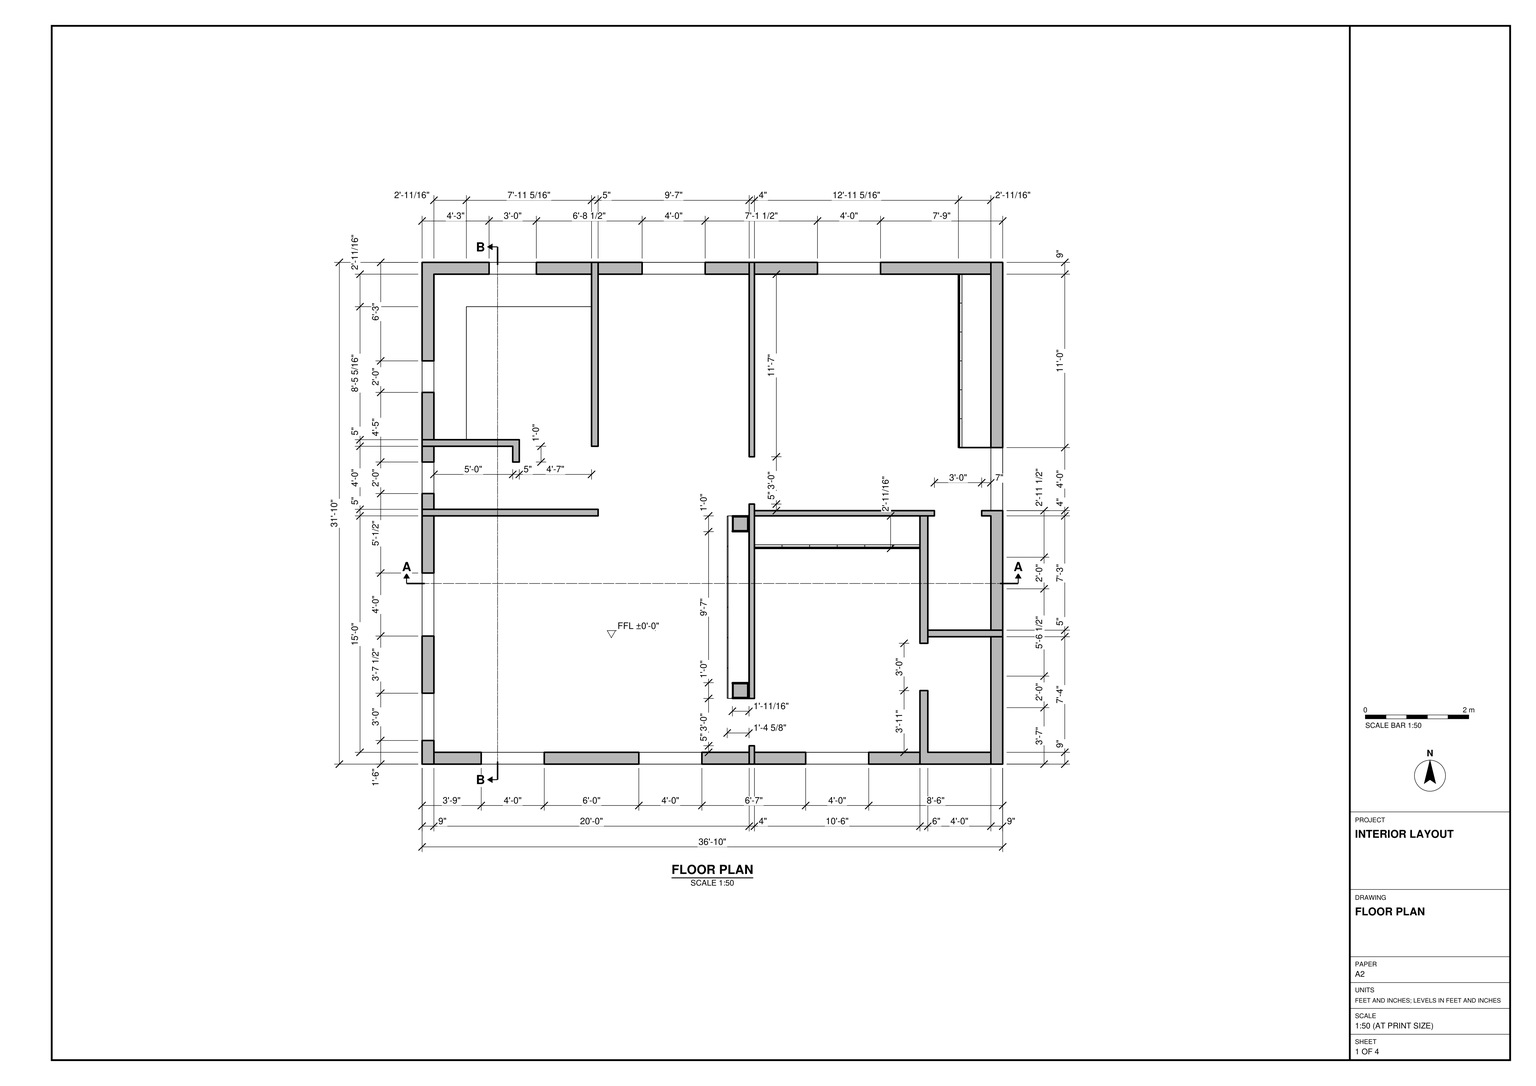
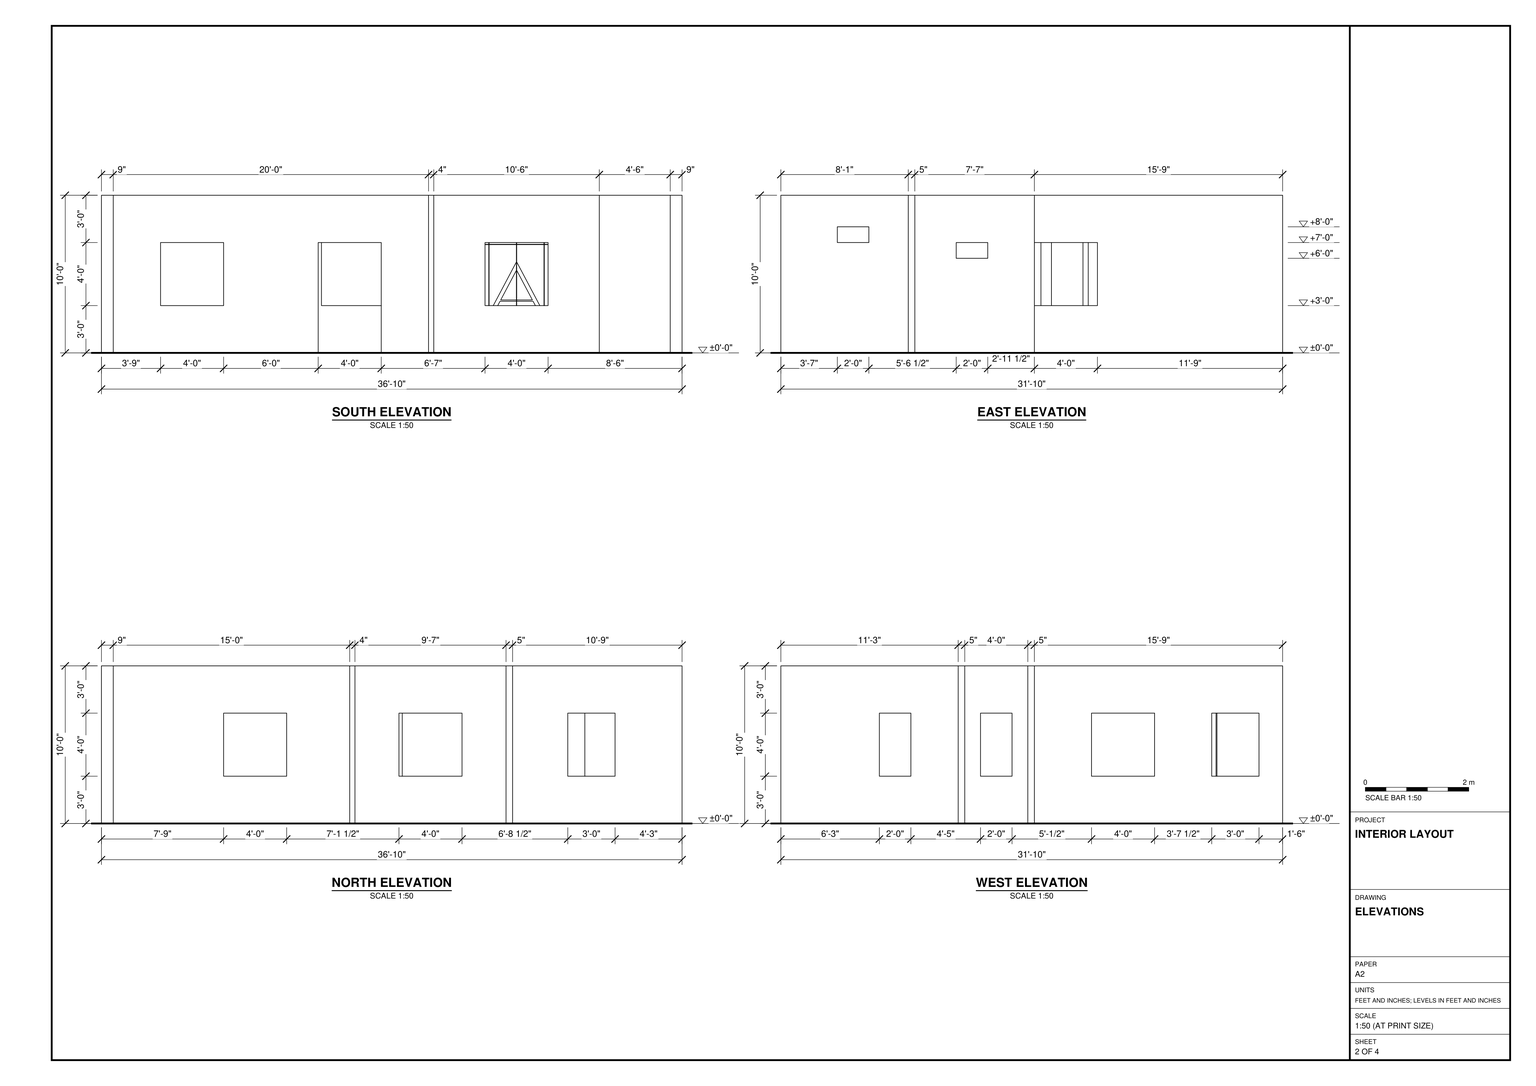
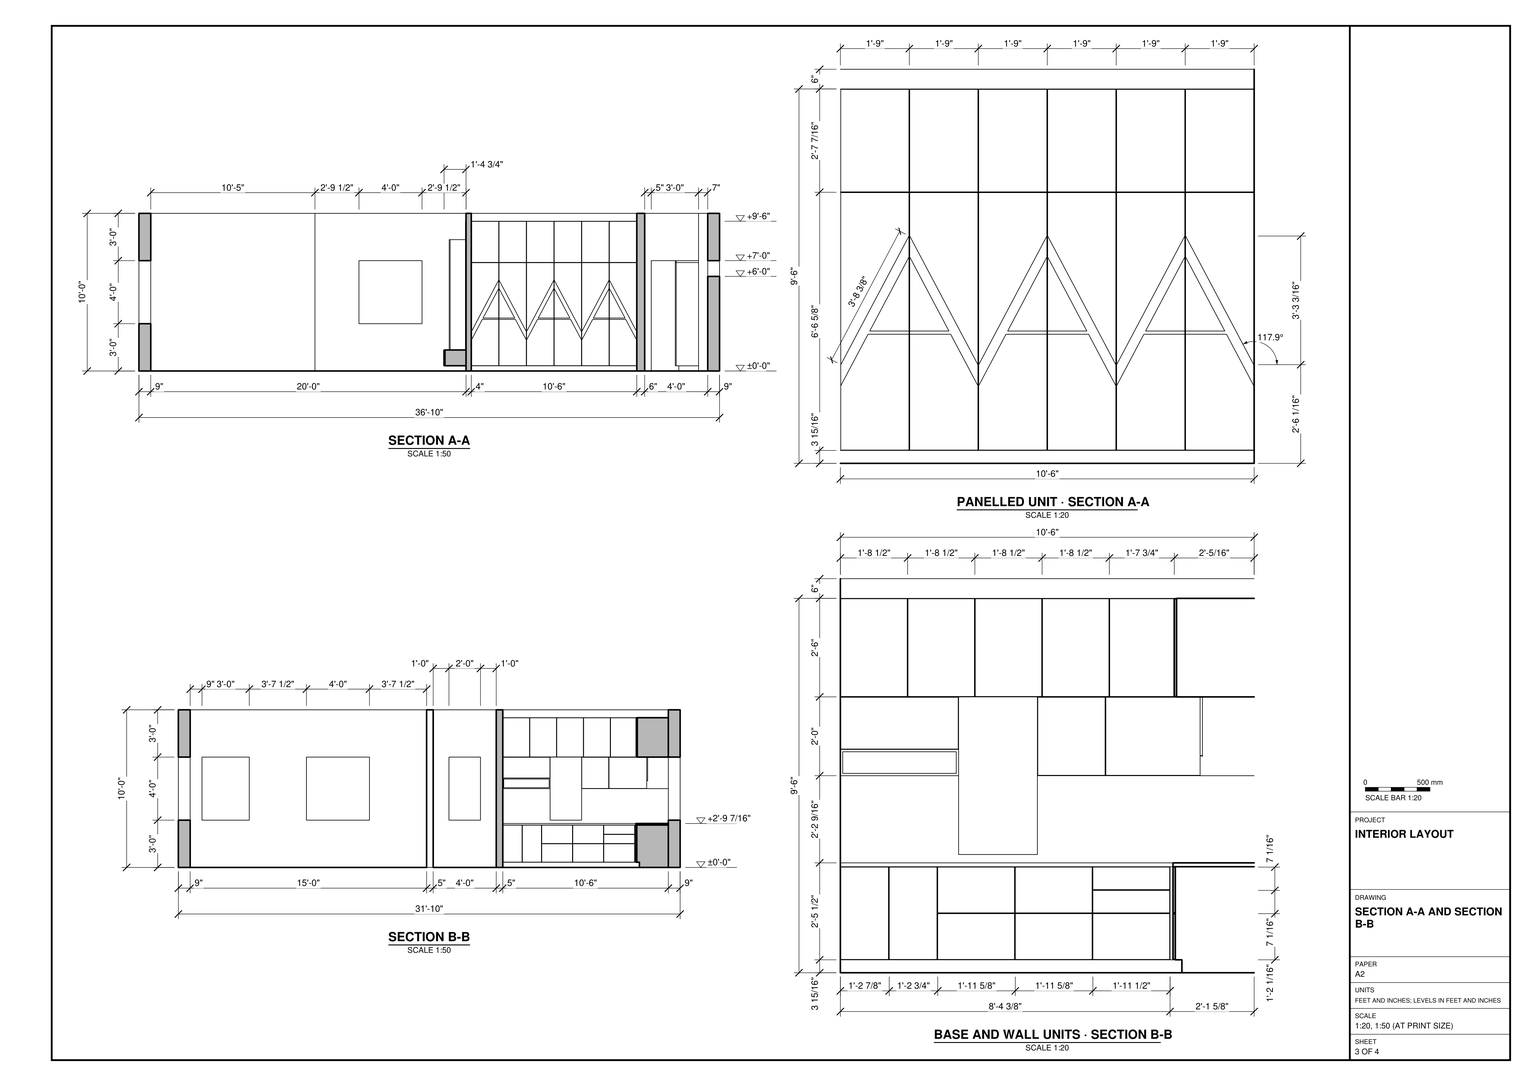
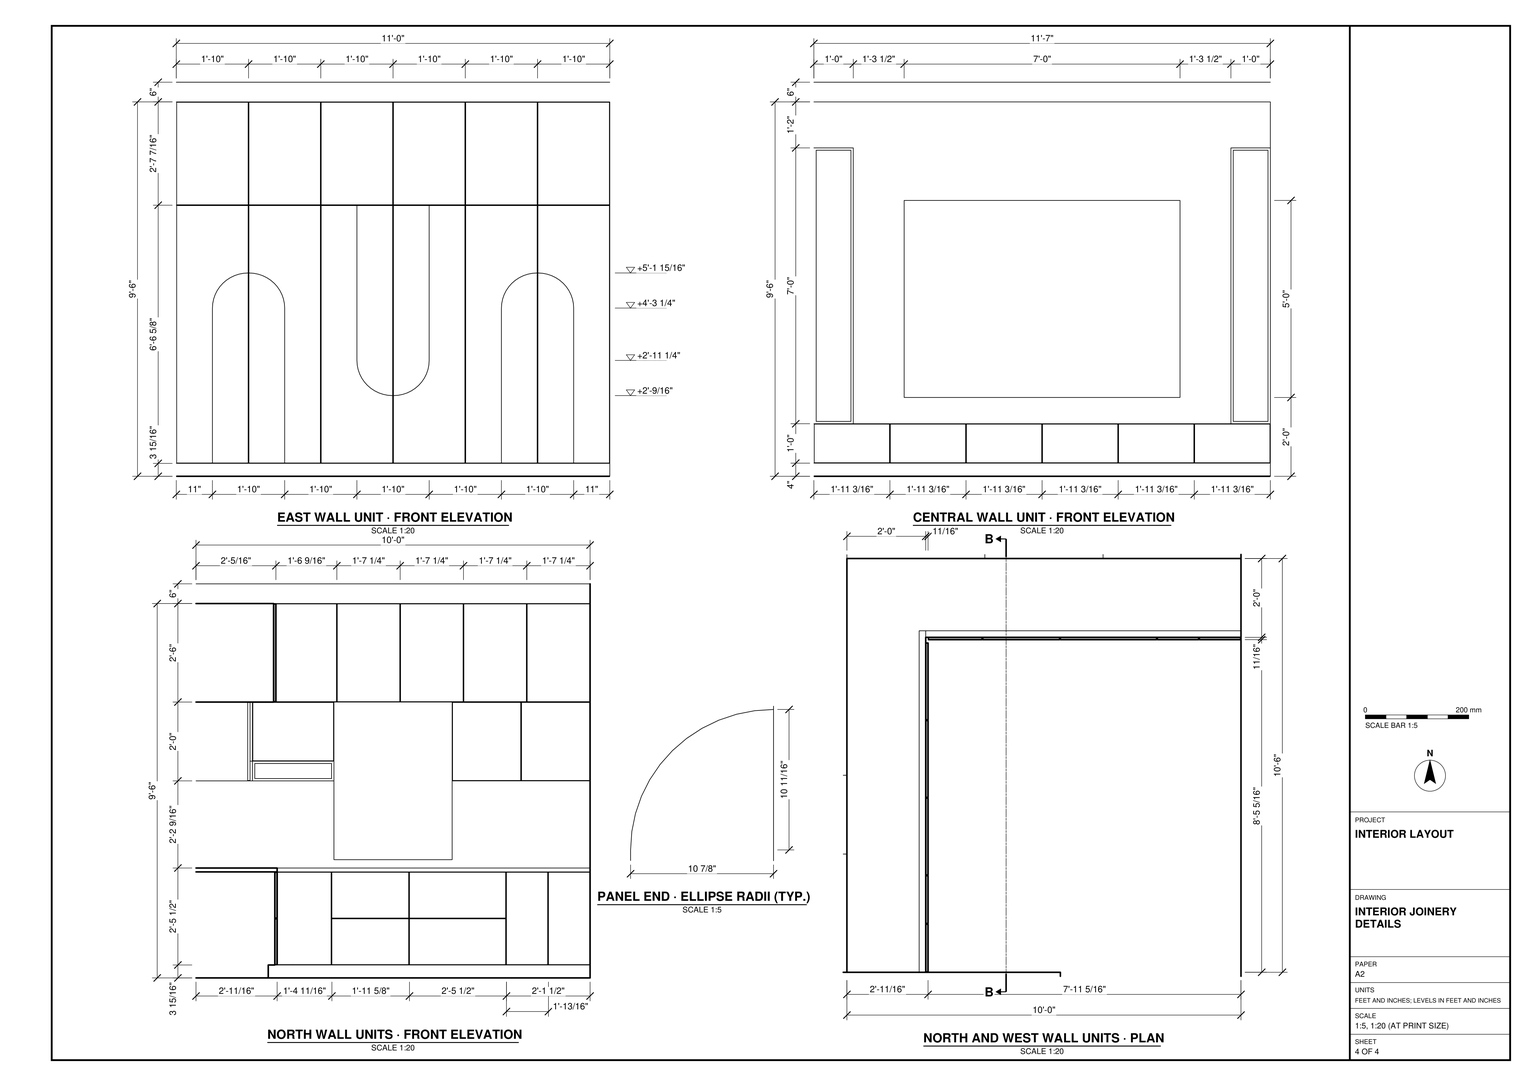
Build the interior in SketchUp using task_files/diagram_01.pdf. Work in feet and inches. Set the finished floor at ±0'-0" and lay out the rectangular shell at 36'-10" east to west by 31'-10" north to south, with an overall height of 10'-0".

Use the floor plan to locate the 9" perimeter walls and follow the individual thicknesses shown for the interior partitions. Preserve the passage between the northern bays and the southern rooms, including the short wall returns and the gaps between partition ends. Form the exterior openings through the walls. Use the elevations to set their widths, sills and heads, particularly the two small openings at different heights on the east wall.

Fit the panelled unit between the partitions shown in section A-A. Carry its three peaked motifs across the six vertical panels. For the cabinetry in section B-B, follow the enlarged detail for the base units, counter, upper cupboards and the spaces between them. Keep shell elements and each furniture or joinery piece in separate groups or components, and use components for repeated parts. Decor and loose items shown may be represented by any suitable library components. Save one SketchUp model as output_files/single_storey_interior_with_built_in_cabinetry.skp.

# SketchUp Ruby script. Lengths in inches.
U = 1.inch
M = Sketchup.active_model
def pt(a) = Geom::Point3d.new(a.map { |v| v * U })
def face(e, loops, mat)
  f = e.add_face(loops[0].map { |a| pt(a) })
  loops[1..].each { |l| e.add_face(l.map { |a| pt(a) }).erase! }
  f.material = f.back_material = mat if mat
  f
end
# faces: each face lists its corners as indices into pts; further lists are holes
def faces(e, pts, list, mat = nil) = list.each { |f| face(e, (f[0].is_a?(Array) ? f : [f]).map { |l| l.map { |i| pts[i] } }, mat) }
# xy, xz, yz: faces in a plane at the given z, y or x. An outline is a flat list of corners, or four numbers for a rectangle; further outlines are holes
def ring(l) = l.size == 4 ? [[l[0], l[1]], [l[2], l[1]], [l[2], l[3]], [l[0], l[3]]] : l.each_slice(2).to_a
def flat(e, list, mat, &to3) = list.each { |f| face(e, (f[0].is_a?(Array) ? f : [f]).map { |l| ring(l).map { |u, v| to3.(u, v) } }, mat) }
def xy(e, z, list, mat = nil) = flat(e, list, mat) { |x, y| [x, y, z] }
def xz(e, y, list, mat = nil) = flat(e, list, mat) { |x, z| [x, y, z] }
def yz(e, x, list, mat = nil) = flat(e, list, mat) { |y, z| [x, y, z] }
def lines(e, pts, list) = list.each { |a, b| e.add_line(pt(pts[a]), pt(pts[b])) }
# prism: a flat outline (further loops are holes) pulled along v
def prism(e, loops, v, mat = nil)
  f = face(e, loops, mat); d = Geom::Vector3d.new(v.map { |x| x * U })
  f.pushpull(f.normal.samedirection?(d) ? d.length : -d.length)
end
def box(e, o, s, mat = nil) = prism(e, [[o, [o[0] + s[0], o[1], o[2]], [o[0] + s[0], o[1] + s[1], o[2]], [o[0], o[1] + s[1], o[2]]]], [0, 0, s[2]], mat)
def at(x, y, z, deg = 0) = Geom::Transformation.translation(pt([x, y, z])) * Geom::Transformation.rotation(ORIGIN, Z_AXIS, deg.degrees)
def axes(o, x, y, z) = Geom::Transformation.new([*x, 0, *y, 0, *z, 0, *pt(o).to_a, 1])
def part(name) = M.definitions.add(name)
# library, detail: a bought-in or finely detailed component or shape, given as its bounding box
def library(name, o, s) = part(name).tap { |d| box(d.entities, o, s) }
def detail(e, o, s) = box(e.add_group.entities, o, s)
def put(e, d, t, mat = nil) = e.add_instance(d, t).tap { |i| i.material = mat if mat }
def group(e, t, mat = nil) = e.add_group.tap { |g| g.transformation = t; g.material = mat if mat }.entities
root = M.entities
M.materials.add("[0006_Pink]").color = [206, 155, 164]
M.materials.add("[0009_Linen]").color = [234, 225, 215]
M.materials.add("[0053_Ivory]").color = [255, 255, 240]
M.materials.add("[0128_White]").color = [255, 255, 255]
M.materials.add("[0129_WhiteSmoke]").color = [237, 237, 237]
M.materials.add("[0132_LightGray]").color = [234, 234, 234]
M.materials.add("[Translucent Glass Gray]").color = [128, 128, 128]
M.materials["[Translucent Glass Gray]"].alpha = 0.5
M.materials.add("[Wood Cherry Original]").color = [152, 86, 42]
c1 = part("Group\#22")
xy(c1.entities,0.12,[[0,0.12,0.71,21.88]])
xy(c1.entities,31.88,[[0,0.12,0.71,21.88]])
xz(c1.entities,0.12,[[0,0.12,0.71,31.88]])
xz(c1.entities,21.88,[[0,0.12,0.71,31.88]])
yz(c1.entities,0,[[0.12,0.12,21.88,31.88]])
yz(c1.entities,0.71,[[[0,0,22,32],[0.12,0.12,21.88,31.88]]])
c2 = part("Group\#51")
xy(c2.entities,0.12,[[0.12,0,20.88,0.71]])
xy(c2.entities,31.88,[[0.12,0,20.88,0.71]])
xz(c2.entities,0,[[0.12,0.12,20.88,31.88]])
xz(c2.entities,0.71,[[[0,0,21,32],[0.12,0.12,20.88,31.88]]])
yz(c2.entities,0.12,[[0,0.12,0.71,31.88]])
yz(c2.entities,20.88,[[0,0.12,0.71,31.88]])
c3 = part("Group\#31")
xy(c3.entities,0.12,[[0.12,0,19.16,0.71]])
xy(c3.entities,29.88,[[0.12,0,19.16,0.71]])
xz(c3.entities,0,[[0.12,0.12,19.16,29.88]])
xz(c3.entities,0.71,[[[0,0,19.28,30],[0.12,0.12,19.16,29.88]]])
yz(c3.entities,0.12,[[0,0.12,0.71,29.88]])
yz(c3.entities,19.16,[[0,0.12,0.71,29.88]])
c4 = part("Group\#32")
xy(c4.entities,0.12,[[0,0.12,0.71,20.36]])
xy(c4.entities,29.88,[[0,0.12,0.71,20.36]])
xz(c4.entities,0.12,[[0,0.12,0.71,29.88]])
xz(c4.entities,20.36,[[0,0.12,0.71,29.88]])
yz(c4.entities,0,[[[0,0,20.48,30],[0.12,0.12,20.36,29.88]]])
yz(c4.entities,0.71,[[0.12,0.12,20.36,29.88]])
c5 = part("Group\#38")
xy(c5.entities,0,[[0,0,12,12]])
xy(c5.entities,0.71,[[0,0.71,11,11.29]])
xy(c5.entities,14.47,[[0,0.71,11,11.29]])
xy(c5.entities,15.18,[[0,0.71,11,11.29]])
xy(c5.entities,28.24,[[0,0.71,11,11.29]])
xy(c5.entities,28.94,[[0,0.71,11,11.29]])
xy(c5.entities,42,[[0,0.71,11,11.29]])
xy(c5.entities,42.71,[[0,0.71,11,11.29]])
xy(c5.entities,55.76,[[0,0.71,11,11.29]])
xy(c5.entities,56.47,[[0,0.71,11,11.29]])
xy(c5.entities,69.53,[[0,0.71,11,11.29]])
xy(c5.entities,70.24,[[0,0.71,11,11.29]])
xy(c5.entities,83.29,[[0,0.71,11,11.29]])
xy(c5.entities,84,[[0,0,12,12]])
xz(c5.entities,0,[[0,0,12,84]])
xz(c5.entities,0.71,[[0,0.71,11,14.47],[0,15.18,11,28.24],[0,28.94,11,42],[0,42.71,11,55.76],[0,56.47,11,69.53],
  [0,70.24,11,83.29]])
xz(c5.entities,11.29,[[0,0.71,11,14.47],[0,15.18,11,28.24],[0,28.94,11,42],[0,42.71,11,55.76],[0,56.47,11,69.53],
  [0,70.24,11,83.29]])
xz(c5.entities,12,[[0,0,12,84]])
yz(c5.entities,0,[[[0,0,12,84],[0.71,0.71,11.29,83.29]],[0.71,14.47,11.29,15.18],[0.71,28.24,11.29,28.94],[0.71,42,11.29,42.71],[0.71,55.76,11.29,56.47],
  [0.71,69.53,11.29,70.24]])
yz(c5.entities,11,[[0.71,0.71,11.29,14.47],[0.71,15.18,11.29,28.24],[0.71,28.94,11.29,42],[0.71,42.71,11.29,55.76],[0.71,56.47,11.29,69.53],
  [0.71,70.24,11.29,83.29]])
yz(c5.entities,12,[[0,0,12,84]])
g1 = group(c5.entities,at(-0.71,0,0))
prism(g1,[[[0.71,0,0],[0.71,12,0],[0.71,12,84],[0.71,0,84]],[[0.71,11.29,0.71],[0.71,0.71,0.71],[0.71,0.71,83.29],[0.71,11.29,83.29]]],[-0.71,0,0])
g2 = group(g1,at(0.2,0.71,0.71),"[Translucent Glass Gray]")
box(g2,[0,0,0],[0.31,10.58,82.58])
c6 = part("Group\#41")
xy(c6.entities,0.12,[[0,0.12,0.71,23.05]])
xy(c6.entities,11.88,[[0,0.12,0.71,23.05]])
xz(c6.entities,0.12,[[0,0.12,0.71,11.88]])
xz(c6.entities,23.05,[[0,0.12,0.71,11.88]])
yz(c6.entities,0,[[0.12,0.12,23.05,11.88]])
yz(c6.entities,0.71,[[[0,0,23.17,12],[0.12,0.12,23.05,11.88]]])
xy(root,0,[[45,0,93,9],[129,0,165,9],[165,0,225,9],[292,0,340,9],[9,9,249,9,249,14,253,14,253,9,379,9,379,56,385,56,385,9,433,9,433,97,385,97,385,92,379,92,379,189,253,189,253,50,249,50,249,198,253,198,253,193,390,193,390,189,385,189,385,102,433,102,433,189,426,189,426,193,433,193,433,373,253,373,253,234,249,234,249,373,134,373,134,242,129,242,129,373,9,373,9,247,74,247,74,230,69,230,69,242,9,242,9,194,134,194,134,189,9,189],
  [0,18,9,54],[433,43,442,67],[0,97.5,9,145.5],[433,133.5,442,157.5],[433,193,442,241],
  [0,206,9,230],[0,283,9,307],[51,373,87,382],[167.5,373,215.5,382],[301,373,349,382]])
xy(root,120,[[0,189,134,194]],"[0132_LightGray]")
xz(root,189,[[0,0,134,120]],"[0132_LightGray]")
xz(root,194,[[0,0,9,120],[9,0,134,120]])
yz(root,0,[[189,0,194,120]],"[0132_LightGray]")
yz(root,134,[[189,0,194,120]])
g3 = group(root,at(0,247,0),"[0132_LightGray]")
xy(g3,0,[[0,0,9,36],[0,36,9,135],[9,126,87,135],[87,126,129,135]])
xy(g3,36,[[0,36,9,60],[51,126,87,135]])
xy(g3,84,[[0,36,9,60],[51,126,87,135]])
xy(g3,120,[[0,0,9,0,9,126,129,126,129,135,0,135]])
xz(g3,0,[[0,0,9,120]])
xz(g3,36,[[0,36,9,84]])
xz(g3,60,[[0,36,9,84]])
xz(g3,126,[[[9,0,129,120],[51,36,87,84]]])
xz(g3,135,[[[0,0,129,120],[51,36,87,84]]])
yz(g3,0,[[[0,0,135,120],[36,36,60,84]]])
yz(g3,9,[[[0,0,126,120],[36,36,60,84]]])
yz(g3,51,[[126,36,135,84]])
yz(g3,87,[[126,36,135,84]])
yz(g3,129,[[126,0,135,120]])
g4 = group(root,at(0,230,0),"[0132_LightGray]")
xy(g4,0,[[69,0,69,12,0,12,0,17,74,17,74,0]])
xy(g4,84,[[69,-36,74,0]])
xy(g4,120,[[69,-36,74,-36,74,17,0,17,0,12,69,12]])
xz(g4,-36,[[69,84,74,120]])
xz(g4,0,[[69,0,74,84]])
xz(g4,12,[[0,0,69,120]])
xz(g4,17,[[0,0,9,120],[9,0,74,120]])
yz(g4,0,[[12,0,17,120]])
yz(g4,69,[[0,0,0,84,-36,84,-36,120,12,120,12,0]])
yz(g4,74,[[0,0,17,0,17,120,-36,120,-36,84,0,84]])
g5 = group(root,at(0,194,0),"[0132_LightGray]")
prism(g5,[[[9,48,120],[9,0,120],[9,0,0],[9,12,0],[9,48,0]],[[9,12,36],[9,12,84],[9,36,84],[9,36,36]]],[-9,0,0])
g6 = group(root,at(0,0,0),"[0132_LightGray]")
prism(g6,[[[9,0,0],[9,18,0],[9,97.5,0],[9,189,0],[9,189,120],[9,0,120]],[[9,97.5,36],[9,97.5,84],[9,145.5,84],[9,145.5,36]],[[9,54,36],[9,18,36],[9,18,84],[9,54,84]]],[-9,0,0])
g7 = group(root,at(9,0,0),"[0132_LightGray]")
prism(g7,[[[240,9,0],[204,9,0],[204,9,84],[156,9,84],[156,9,0],[84,9,0],[0,9,0],[0,9,120],[240,9,120]],[[36,9,36],[84,9,36],[84,9,84],[36,9,84]]],[0,-9,0])
g8 = group(root,at(249,0,0),"[0132_LightGray]")
xy(g8,0,[[0,0,4,14],[0,50,4,198]])
xy(g8,84,[[0,14,4,50]])
xy(g8,120,[[0,0,4,198]])
xz(g8,0,[[0,0,4,120]])
xz(g8,14,[[0,0,4,84]])
xz(g8,50,[[0,0,4,84]])
xz(g8,198,[[0,0,4,120]])
yz(g8,0,[[0,0,9,120],[9,0,9,120,198,120,198,0,50,0,50,84,14,84,14,0]])
yz(g8,4,[[0,0,14,0,14,84,50,84,50,0,198,0,198,120,0,120]])
g9 = group(root,at(253,0,0),"[0132_LightGray]")
prism(g9,[[[126,9,0],[87,9,0],[0,9,0],[0,9,120],[126,9,120]],[[39,9,36],[87,9,36],[87,9,84],[39,9,84]]],[0,-9,0])
g10 = group(root,at(379,0,0),"[0132_LightGray]")
xy(g10,0,[[0,0,6,56],[6,0,54,9]])
xy(g10,84,[[0,56,6,92]])
xy(g10,120,[[0,0,54,0,54,9,6,9,6,92,0,92]])
xz(g10,0,[[0,0,54,120]])
xz(g10,9,[[6,0,54,120]])
xz(g10,56,[[0,0,6,84]])
xz(g10,92,[[0,84,6,120]])
yz(g10,0,[[0,0,9,120],[9,0,9,120,92,120,92,84,56,84,56,0]])
yz(g10,6,[[9,0,56,0,56,84,92,84,92,120,9,120]])
yz(g10,54,[[0,0,9,120]])
g11 = group(root,at(433,0,0),"[0132_LightGray]")
xy(g11,0,[[0,0,9,67],[0,67,9,97]])
xy(g11,84,[[0,43,9,67]])
xy(g11,96,[[0,43,9,67]])
xy(g11,120,[[0,0,9,97]])
xz(g11,0,[[0,0,9,120]])
xz(g11,43,[[0,84,9,96]])
xz(g11,67,[[0,84,9,96]])
xz(g11,97,[[0,0,9,120]])
yz(g11,0,[[0,0,9,120],[[9,0,97,120],[43,84,67,96]]])
yz(g11,9,[[[0,0,97,120],[43,84,67,96]]])
g12 = group(root,at(385,97,0),"[0132_LightGray]")
prism(g12,[[[48,0,0],[0,0,0],[0,5,0],[57,5,0],[57,0,0]]],[0,0,120])
g13 = group(root,at(426,102,0),"[0132_LightGray]")
xy(g13,0,[[7,0,16,55.5],[7,55.5,7,87,0,87,0,91,16,91,16,55.5]])
xy(g13,72,[[7,31.5,16,55.5]])
xy(g13,84,[[7,31.5,16,55.5]])
xy(g13,120,[[7,0,16,0,16,91,0,91,0,87,7,87]])
xz(g13,0,[[7,0,16,120]])
xz(g13,31.5,[[7,72,16,84]])
xz(g13,55.5,[[7,72,16,84]])
xz(g13,87,[[0,0,7,120]])
xz(g13,91,[[0,0,16,120]])
yz(g13,0,[[87,0,91,120]])
yz(g13,7,[[[0,0,87,120],[31.5,72,55.5,84]]])
yz(g13,16,[[[0,0,91,120],[31.5,72,55.5,84]]])
g14 = group(root,at(379,92,0),"[0132_LightGray]")
prism(g14,[[[0,0,0],[0,97,0],[6,97,0],[6,10,0],[6,5,0],[6,0,0]]],[0,0,120])
g15 = group(root,at(253,189,0),"[0132_LightGray]")
xy(g15,0,[[0,0,137,4]])
xy(g15,84,[[137,0,173,4]])
xy(g15,120,[[0,0,173,4]])
xz(g15,0,[[0,0,126,120],[126,0,132,120],[132,0,137,0,137,84,173,84,173,120,132,120]])
xz(g15,4,[[0,0,0,120,173,120,173,84,137,84,137,0]])
yz(g15,0,[[0,0,4,120]])
yz(g15,137,[[0,0,4,84]])
yz(g15,173,[[0,84,4,120]])
g16 = group(root,at(433,241,0),"[0132_LightGray]")
prism(g16,[[[0,-48,84],[0,-48,120],[0,141,120],[0,141,0],[0,-48,0],[0,-48,36],[0,0,36],[0,0,84]]],[9,0,0])
g17 = group(root,at(129,242,0),"[0132_LightGray]")
prism(g17,[[[5,140,0],[5,0,0],[0,0,0],[0,131,0],[0,140,0]]],[0,0,120])
g18 = group(root,at(134,373,0),"[0132_LightGray]")
prism(g18,[[[115,0,0],[115,0,120],[0,0,120],[0,0,0],[33.5,0,0]],[[33.5,0,36],[33.5,0,84],[81.5,0,84],[81.5,0,36]]],[0,9,0])
g19 = group(root,at(249,234,0),"[0132_LightGray]")
xy(g19,0,[[0,0,4,148]])
xy(g19,84,[[0,-36,4,0]])
xy(g19,120,[[0,-36,4,148]])
xz(g19,-36,[[0,84,4,120]])
xz(g19,0,[[0,0,4,84]])
xz(g19,148,[[0,0,4,120]])
yz(g19,0,[[0,0,0,84,-36,84,-36,120,139,120,139,0],[139,0,148,120]])
yz(g19,4,[[0,0,148,0,148,120,-36,120,-36,84,0,84]])
g20 = group(root,at(253,373,0),"[0132_LightGray]")
prism(g20,[[[180,9,0],[96,9,0],[0,9,0],[0,9,120],[180,9,120]],[[48,9,36],[96,9,36],[96,9,84],[48,9,84]]],[0,-9,0])
g21 = group(root,at(409,234,0),"[0009_Linen]")
xy(g21,0,[[2,7,24,139]])
xy(g21,3.93,[[0,7,2,29],[2,7,24,139],[0,29,2,51],[0,51,2,73],[0,73,2,95],
  [0,95,2,117],[0,117,2,139]])
xy(g21,82.55,[[0,7,24,139]])
xy(g21,114,[[0,7,24,139]])
xz(g21,7,[[2,0,24,3.93],[0,3.93,24,82.55],[0,82.55,24,114]])
xz(g21,139,[[2,0,24,3.93],[0,3.93,24,82.55],[0,82.55,24,114]])
yz(g21,0,[[7,3.93,29,82.55],[29,3.93,51,82.55],[51,3.93,73,82.55],[73,3.93,95,82.55],[95,3.93,117,82.55],
  [117,3.93,139,82.55],[7,82.55,29,114],[29,82.55,51,114],[51,82.55,73,114],[73,82.55,95,114],
  [95,82.55,117,114],[117,82.55,139,114]])
yz(g21,2,[[7,0,139,3.93]])
yz(g21,24,[[7,0,139,3.93],[7,3.93,139,82.55],[7,82.55,139,114]])
g22 = group(g21,at(-0.71,29,3.93))
xy(g22,0.12,[[0,0.12,0.71,21.88]])
xy(g22,78.5,[[0,0.12,0.71,21.88]])
xz(g22,0.12,[[0,0.12,0.71,78.5]])
xz(g22,21.88,[[0,0.12,0.71,78.5]])
yz(g22,0,[[11,0.12,11,47.29,10.91,48.68,10.63,50.06,10.17,51.38,9.54,52.64,8.75,53.8,7.8125,54.85,6.74,55.77,5.56,56.55,4.28,57.17,2.93,57.62,1.54,57.89,0.12,57.98,0.12,78.5,21.88,78.5,21.88,0.12]])
yz(g22,0,[[0.12,0.12,0.12,57.98,1.54,57.89,2.93,57.62,4.28,57.17,5.56,56.55,6.74,55.77,7.8125,54.85,8.75,53.8,9.54,52.64,10.17,51.38,10.63,50.06,10.91,48.68,11,47.29,11,0.12]],"[0129_WhiteSmoke]")
yz(g22,0.71,[[[0,0,22,78.62],[0.12,0.12,21.88,78.5]]])
g23 = group(g21,at(-0.71,29,3.93))
xy(g23,0.12,[[0,-21.88,0.71,-0.12]])
xy(g23,78.5,[[0,-21.88,0.71,-0.12]])
xz(g23,-21.88,[[0,0.12,0.71,78.5]])
xz(g23,-0.12,[[0,0.12,0.71,78.5]])
yz(g23,0,[[-21.88,0.12,-11,0.12,-11,47.29,-10.91,48.68,-10.63,50.06,-10.17,51.38,-9.54,52.64,-8.75,53.8,-7.8125,54.85,-6.74,55.77,-5.56,56.55,-4.28,57.17,-2.93,57.62,-1.54,57.89,-0.12,57.98,-0.12,78.5,-21.88,78.5]])
yz(g23,0,[[-11,0.12,-0.12,0.12,-0.12,57.98,-1.54,57.89,-2.93,57.62,-4.28,57.17,-5.56,56.55,-6.74,55.77,-7.8125,54.85,-8.75,53.8,-9.54,52.64,-10.17,51.38,-10.63,50.06,-10.91,48.68,-11,47.29]],"[0129_WhiteSmoke]")
yz(g23,0.71,[[[-22,0,0,78.62],[-21.88,0.12,-0.12,78.5]]])
g24 = group(g21,at(-0.71,117,3.93))
xy(g24,0.12,[[0,-21.88,0.71,-0.12]])
xy(g24,78.5,[[0,-21.88,0.71,-0.12]])
xz(g24,-21.88,[[0,0.12,0.71,78.5]])
xz(g24,-0.12,[[0,0.12,0.71,78.5]])
yz(g24,0,[[-21.88,0.12,-11,0.12,-11,47.29,-10.91,48.68,-10.63,50.06,-10.17,51.38,-9.54,52.64,-8.75,53.8,-7.8125,54.85,-6.74,55.77,-5.56,56.55,-4.28,57.17,-2.93,57.62,-1.54,57.89,-0.12,57.98,-0.12,78.5,-21.88,78.5]])
yz(g24,0,[[-11,0.12,-0.12,0.12,-0.12,57.98,-1.54,57.89,-2.93,57.62,-4.28,57.17,-5.56,56.55,-6.74,55.77,-7.8125,54.85,-8.75,53.8,-9.54,52.64,-10.17,51.38,-10.63,50.06,-10.91,48.68,-11,47.29]],"[0129_WhiteSmoke]")
yz(g24,0.71,[[[-22,0,0,78.62],[-21.88,0.12,-0.12,78.5]]])
g25 = group(g21,at(-0.71,117,3.93))
xy(g25,0.12,[[0,0.12,0.71,21.88]])
xy(g25,78.5,[[0,0.12,0.71,21.88]])
xz(g25,0.12,[[0,0.12,0.71,78.5]])
xz(g25,21.88,[[0,0.12,0.71,78.5]])
yz(g25,0,[[11,0.12,11,47.29,10.91,48.68,10.63,50.06,10.17,51.38,9.54,52.64,8.75,53.8,7.8125,54.85,6.74,55.77,5.56,56.55,4.28,57.17,2.93,57.62,1.54,57.89,0.12,57.98,0.12,78.5,21.88,78.5,21.88,0.12]])
yz(g25,0,[[0.12,0.12,0.12,57.98,1.54,57.89,2.93,57.62,4.28,57.17,5.56,56.55,6.74,55.77,7.8125,54.85,8.75,53.8,9.54,52.64,10.17,51.38,10.63,50.06,10.91,48.68,11,47.29,11,0.12]],"[0129_WhiteSmoke]")
yz(g25,0.71,[[[0,0,22,78.62],[0.12,0.12,21.88,78.5]]])
g26 = group(g21,at(-0.71,73,82.55))
xy(g26,-78.5,[[0,-21.88,0.71,-0.12]])
xy(g26,-0.12,[[0,-21.88,0.71,-0.12]])
xz(g26,-21.88,[[0,-78.5,0.71,-0.12]])
xz(g26,-0.12,[[0,-78.5,0.71,-0.12]])
yz(g26,0,[[-21.88,-78.5,-21.88,-0.12,-11,-0.12,-11,-47.29,-10.91,-48.68,-10.63,-50.06,-10.17,-51.38,-9.54,-52.64,-8.75,-53.8,-7.8125,-54.85,-6.74,-55.77,-5.56,-56.55,-4.28,-57.17,-2.93,-57.62,-1.54,-57.89,-0.12,-57.98,-0.12,-78.5]])
yz(g26,0,[[-0.12,-57.98,-1.54,-57.89,-2.93,-57.62,-4.28,-57.17,-5.56,-56.55,-6.74,-55.77,-7.8125,-54.85,-8.75,-53.8,-9.54,-52.64,-10.17,-51.38,-10.63,-50.06,-10.91,-48.68,-11,-47.29,-11,-0.12,-0.12,-0.12]],"[0129_WhiteSmoke]")
yz(g26,0.71,[[[-22,-78.62,0,0],[-21.88,-78.5,-0.12,-0.12]]])
g27 = group(g21,at(-0.71,73,82.55))
xy(g27,-78.5,[[0,0.12,0.71,21.88]])
xy(g27,-0.12,[[0,0.12,0.71,21.88]])
xz(g27,0.12,[[0,-78.5,0.71,-0.12]])
xz(g27,21.88,[[0,-78.5,0.71,-0.12]])
yz(g27,0,[[0.12,-78.5,21.88,-78.5,21.88,-0.12,11,-0.12,11,-47.29,10.91,-48.68,10.63,-50.06,10.17,-51.38,9.54,-52.64,8.75,-53.8,7.8125,-54.85,6.74,-55.77,5.56,-56.55,4.28,-57.17,2.93,-57.62,1.54,-57.89,0.12,-57.98]])
yz(g27,0,[[0.12,-57.98,1.54,-57.89,2.93,-57.62,4.28,-57.17,5.56,-56.55,6.74,-55.77,7.8125,-54.85,8.75,-53.8,9.54,-52.64,10.17,-51.38,10.63,-50.06,10.91,-48.68,11,-47.29,11,-0.12,0.12,-0.12]],"[0129_WhiteSmoke]")
yz(g27,0.71,[[[0,-78.62,22,0],[0.12,-78.5,21.88,-0.12]]])
put(g21,c1,axes([-0.71,117,82.55],[1,0,0],[0,1,0],[0,0,0.98276]))
put(g21,c1,axes([-0.71,95,82.55],[1,0,0],[0,1,0],[0,0,0.98276]))
put(g21,c1,axes([-0.71,73,82.55],[1,0,0],[0,1,0],[0,0,0.98276]))
put(g21,c1,axes([-0.71,51,82.55],[1,0,0],[0,1,0],[0,0,0.98276]))
put(g21,c1,axes([-0.71,29,82.55],[1,0,0],[0,1,0],[0,0,0.98276]))
put(g21,c1,axes([-0.71,7,82.55],[1,0,0],[0,1,0],[0,0,0.98276]))
g28 = group(root,at(253,165,0),"[0006_Pink]")
xy(g28,0,[[0,2,126,24]])
xy(g28,3.93,[[0,0,21,2],[21,0,42,2],[42,0,63,2],[63,0,84,2],[84,0,105,2],
  [105,0,126,2],[0,2,126,24]])
xy(g28,82.55,[[0,0,126,24]])
xy(g28,114,[[0,0,126,24]])
xz(g28,0,[[0,3.93,21,82.55],[21,3.93,42,82.55],[42,3.93,63,82.55],[63,3.93,84,82.55],[84,3.93,105,82.55],
  [105,3.93,126,82.55],[0,82.55,21,114],[21,82.55,42,114],[42,82.55,63,114],[63,82.55,84,114],
  [84,82.55,105,114],[105,82.55,126,114]])
xz(g28,2,[[0,0,126,3.93]])
xz(g28,24,[[0,0,126,3.93],[0,3.93,126,82.55],[0,82.55,126,114]])
yz(g28,0,[[2,0,24,3.93],[0,3.93,24,82.55],[0,82.55,24,114]])
yz(g28,126,[[2,0,24,3.93],[0,3.93,24,82.55],[0,82.55,24,114]])
g29 = group(g28,at(0,-0.71,3.93))
xy(g29,0.12,[[0.12,0,20.88,0.71]])
xy(g29,78.5,[[0.12,0,20.88,0.71]])
xz(g29,0,[[0.12,0.12,20.88,0.12,20.88,35.38,8.42,35.38,0.12,19.71],[0.12,26.1,5.76,36.74,20.88,65.29,20.88,78.5,0.12,78.5],[8.9375,36.36,20.88,36.36,20.88,58.91]])
xz(g29,0,[[0.12,19.71,8.42,35.38,20.88,35.38,20.88,36.36,8.9375,36.36,20.88,58.91,20.88,65.29,5.76,36.74,0.12,26.1]],"[0128_White]")
xz(g29,0.71,[[[0,0,21,78.62],[0.12,0.12,20.88,78.5]]])
yz(g29,0.12,[[0,0.12,0.71,78.5]])
yz(g29,20.88,[[0,0.12,0.71,78.5]])
g30 = group(g28,at(42,-0.71,3.93))
xy(g30,0.12,[[-20.88,0,-0.12,0.71]])
xy(g30,78.5,[[-20.88,0,-0.12,0.71]])
xz(g30,0,[[-20.88,0.12,-20.88,35.38,-8.42,35.38,-0.12,19.71,-0.12,0.12],[-0.12,26.1,-5.76,36.74,-20.88,65.29,-20.88,78.5,-0.12,78.5],[-20.88,36.36,-20.88,58.91,-8.9375,36.36]])
xz(g30,0,[[-0.12,19.71,-8.42,35.38,-20.88,35.38,-20.88,36.36,-8.9375,36.36,-20.88,58.91,-20.88,65.29,-5.76,36.74,-0.12,26.1]],"[0128_White]")
xz(g30,0.71,[[[-21,0,0,78.62],[-20.88,0.12,-0.12,78.5]]])
yz(g30,-20.88,[[0,0.12,0.71,78.5]])
yz(g30,-0.12,[[0,0.12,0.71,78.5]])
g31 = group(g28,at(126,-0.71,3.93))
xy(g31,0.12,[[-20.88,0,-0.12,0.71]])
xy(g31,78.5,[[-20.88,0,-0.12,0.71]])
xz(g31,0,[[-20.88,0.12,-20.88,35.38,-8.42,35.38,-0.12,19.71,-0.12,0.12],[-0.12,26.1,-5.76,36.74,-20.88,65.29,-20.88,78.5,-0.12,78.5],[-20.88,36.36,-20.88,58.91,-8.9375,36.36]])
xz(g31,0,[[-0.12,19.71,-8.42,35.38,-20.88,35.38,-20.88,36.36,-8.9375,36.36,-20.88,58.91,-20.88,65.29,-5.76,36.74,-0.12,26.1]],"[0128_White]")
xz(g31,0.71,[[[-21,0,0,78.62],[-20.88,0.12,-0.12,78.5]]])
yz(g31,-20.88,[[0,0.12,0.71,78.5]])
yz(g31,-0.12,[[0,0.12,0.71,78.5]])
g32 = group(g28,at(84,-0.71,3.93))
xy(g32,0.12,[[0.12,0,20.88,0.71]])
xy(g32,78.5,[[0.12,0,20.88,0.71]])
xz(g32,0,[[0.12,0.12,20.88,0.12,20.88,35.38,8.42,35.38,0.12,19.71],[0.12,26.1,5.76,36.74,20.88,65.29,20.88,78.5,0.12,78.5],[8.9375,36.36,20.88,36.36,20.88,58.91]])
xz(g32,0,[[0.12,19.71,8.42,35.38,20.88,35.38,20.88,36.36,8.9375,36.36,20.88,58.91,20.88,65.29,5.76,36.74,0.12,26.1]],"[0128_White]")
xz(g32,0.71,[[[0,0,21,78.62],[0.12,0.12,20.88,78.5]]])
yz(g32,0.12,[[0,0.12,0.71,78.5]])
yz(g32,20.88,[[0,0.12,0.71,78.5]])
g33 = group(g28,at(84,-0.71,3.93))
xy(g33,0.12,[[-20.88,0,-0.12,0.71]])
xy(g33,78.5,[[-20.88,0,-0.12,0.71]])
xz(g33,0,[[-0.12,19.71,-8.42,35.38,-20.88,35.38,-20.88,36.36,-8.9375,36.36,-20.88,58.91,-20.88,65.29,-5.76,36.74,-0.12,26.1]],"[0006_Pink]")
xz(g33,0,[[-20.88,0.12,-20.88,35.38,-8.42,35.38,-0.12,19.71,-0.12,0.12],[-0.12,26.1,-5.76,36.74,-20.88,65.29,-20.88,78.5,-0.12,78.5],[-20.88,36.36,-20.88,58.91,-8.9375,36.36]],"[0128_White]")
xz(g33,0.71,[[[-21,0,0,78.62],[-20.88,0.12,-0.12,78.5]]])
yz(g33,-20.88,[[0,0.12,0.71,78.5]])
yz(g33,-0.12,[[0,0.12,0.71,78.5]])
g34 = group(g28,at(42,-0.71,3.93))
xy(g34,0.12,[[0.12,0,20.88,0.71]])
xy(g34,78.5,[[0.12,0,20.88,0.71]])
xz(g34,0,[[0.12,19.71,8.42,35.38,20.88,35.38,20.88,36.36,8.9375,36.36,20.88,58.91,20.88,65.29,5.76,36.74,0.12,26.1]])
xz(g34,0,[[0.12,0.12,20.88,0.12,20.88,35.38,8.42,35.38,0.12,19.71],[0.12,26.1,5.76,36.74,20.88,65.29,20.88,78.5,0.12,78.5],[8.9375,36.36,20.88,36.36,20.88,58.91]],"[0128_White]")
xz(g34,0.71,[[[0,0,21,78.62],[0.12,0.12,20.88,78.5]]])
yz(g34,0.12,[[0,0.12,0.71,78.5]])
yz(g34,20.88,[[0,0.12,0.71,78.5]])
g35 = group(g28,at(0,-0.71,82.55),"[0006_Pink]")
xy(g35,0.12,[[0.12,0,20.88,0.71]],"[0006_Pink]")
xy(g35,31.33,[[0.12,0,20.88,0.71]],"[0006_Pink]")
xz(g35,0,[[0.12,0.12,20.88,31.33]],"[0006_Pink]")
xz(g35,0.71,[[[0,0,21,31.45],[0.12,0.12,20.88,31.33]]],"[0006_Pink]")
yz(g35,0.12,[[0,0.12,0.71,31.33]],"[0006_Pink]")
yz(g35,20.88,[[0,0.12,0.71,31.33]],"[0006_Pink]")
put(g28,c2,axes([21,-0.71,82.55],[1,0,0],[0,1,0],[0,0,0.98276]),"[0006_Pink]")
g36 = group(g28,at(42,-0.71,82.55))
xy(g36,0.12,[[0.12,0,20.88,0.71]])
xy(g36,31.33,[[0.12,0,20.88,0.71]])
xz(g36,0,[[0.12,0.12,20.88,31.33]])
xz(g36,0.71,[[[0,0,21,31.45],[0.12,0.12,20.88,31.33]]])
yz(g36,0.12,[[0,0.12,0.71,31.33]])
yz(g36,20.88,[[0,0.12,0.71,31.33]])
put(g28,c2,axes([63,-0.71,82.55],[1,0,0],[0,1,0],[0,0,0.98276]))
put(g28,c2,axes([84,-0.71,82.55],[1,0,0],[0,1,0],[0,0,0.98276]),"[0006_Pink]")
put(g28,c2,axes([105,-0.71,82.55],[1,0,0],[0,1,0],[0,0,0.98276]),"[0006_Pink]")
g37 = group(root,at(9,247,0),"[0053_Ivory]")
xy(g37,0,[[0,0,0,126,120,126,120,104,22,104,22,0]])
xy(g37,3.9375,[[22,0,24,104],[24,102,120,104]])
xy(g37,32.28,[[0,0,0,126,120,126,120,102,24,102,24,0],[24,0,24.71,29.53],[24,29.53,24.71,53.15],[24,53.15,24.71,76.77],[24,76.77,24.71,100.39],
  [24,100.39,24.71,101.29],[24,101.29,29.45,102],[29.45,101.29,41.26,102],[41.26,101.29,64.88,102],[64.88,101.29,94.41,102],
  [94.41,101.29,120,102]])
xy(g37,33.46,[[0,0,24.71,0,24.71,101.29,120,101.29,120,126,0,126]])
xz(g37,0,[[0,0,22,0,22,3.9375,24,3.9375,24,32.28,0,32.28],[0,32.28,24.71,33.46]])
xz(g37,101.29,[[24.71,32.28,120,33.46]])
xz(g37,102,[[24,3.9375,29.45,32.28],[29.45,3.9375,41.26,32.28],[41.26,3.9375,64.88,32.28],[64.88,3.9375,94.41,32.28],[94.41,3.9375,120,32.28]])
xz(g37,104,[[22,0,120,3.9375]])
xz(g37,126,[[0,0,120,32.28],[0,32.28,120,33.46]])
yz(g37,0,[[0,0,126,32.28],[0,32.28,126,33.46]])
yz(g37,22,[[0,0,104,3.9375]])
yz(g37,24,[[0,3.9375,29.53,32.28],[29.53,3.9375,53.15,32.28],[53.15,3.9375,76.77,32.28],[76.77,3.9375,100.39,32.28],[100.39,3.9375,102,32.28]])
yz(g37,24.71,[[0,32.28,101.29,33.46]])
yz(g37,120,[[104,0,126,0,126,32.28,102,32.28,102,3.9375,104,3.9375],[101.29,32.28,126,33.46]])
g38 = group(g37,at(24,0,3.9375))
xy(g38,0.12,[[0,0.12,0.71,14.65],[0,14.88,0.71,29.41],[0,29.65,0.71,53.03],[0,53.27,0.71,76.65],[0,76.89,0.71,100.28]])
xy(g38,14.06,[[0,29.65,0.71,53.03],[0,53.27,0.71,76.65],[0,76.89,0.71,100.28]])
xy(g38,14.29,[[0,29.65,0.71,53.03],[0,53.27,0.71,76.65],[0,76.89,0.71,100.28]])
xy(g38,21.14,[[0,76.89,0.71,100.28]])
xy(g38,21.38,[[0,76.89,0.71,100.28]])
xy(g38,28.23,[[0,0.12,0.71,14.65],[0,14.88,0.71,29.41],[0,29.65,0.71,53.03],[0,53.27,0.71,76.65],[0,76.89,0.71,100.28]])
xz(g38,0.12,[[0,0.12,0.71,28.23]])
xz(g38,14.65,[[0,0.12,0.71,28.23]])
xz(g38,14.88,[[0,0.12,0.71,28.23]])
xz(g38,29.41,[[0,0.12,0.71,14.17],[0,14.17,0.71,28.23]])
xz(g38,29.65,[[0,0.12,0.71,14.06],[0,14.29,0.71,28.23]])
xz(g38,53.03,[[0,0.12,0.71,14.06],[0,14.29,0.71,28.23]])
xz(g38,53.27,[[0,0.12,0.71,14.06],[0,14.29,0.71,28.23]])
xz(g38,76.65,[[0,0.12,0.71,14.06],[0,14.29,0.71,21.26],[0,21.26,0.71,28.23]])
xz(g38,76.89,[[0,0.12,0.71,14.06],[0,14.29,0.71,21.14],[0,21.38,0.71,28.23]])
xz(g38,100.28,[[0,0.12,0.71,14.06],[0,14.29,0.71,21.14],[0,21.38,0.71,28.23]])
yz(g38,0,[[[0,0,14.76,28.35],[0.12,0.12,14.65,28.23]],[[14.76,0,29.53,28.35],[14.88,0.12,29.41,28.23]],[[29.53,0,53.15,14.17],[29.65,0.12,53.03,14.06]],[[53.15,0,76.77,14.17],[53.27,0.12,76.65,14.06]],[[76.77,0,100.39,14.17],[76.89,0.12,100.28,14.06]],
  [[29.53,14.17,53.15,28.35],[29.65,14.29,53.03,28.23]],[[53.15,14.17,76.77,28.35],[53.27,14.29,76.65,28.23]],[[76.77,14.17,100.39,21.26],[76.89,14.29,100.28,21.14]],[[76.77,21.26,100.39,28.35],[76.89,21.38,100.28,28.23]]])
yz(g38,0.71,[[0.12,0.12,14.65,28.23],[14.88,0.12,29.41,28.23],[29.65,0.12,53.03,14.06],[53.27,0.12,76.65,14.06],[76.89,0.12,100.28,14.06],
  [29.65,14.29,53.03,28.23],[53.27,14.29,76.65,28.23],[76.89,14.29,100.28,21.14],[76.89,21.38,100.28,28.23]])
g39 = group(g37,at(24.71,102,3.9375))
xy(g39,0.12,[[0.12,-0.71,16.43,0],[16.67,-0.71,40.06,0],[40.29,-0.71,69.58,0],[69.82,-0.71,82.38,0],[82.61,-0.71,95.17,0]])
xy(g39,14.06,[[16.67,-0.71,40.06,0],[40.29,-0.71,69.58,0]])
xy(g39,14.29,[[16.67,-0.71,40.06,0],[40.29,-0.71,69.58,0]])
xy(g39,28.23,[[0.12,-0.71,16.43,0],[16.67,-0.71,40.06,0],[40.29,-0.71,69.58,0],[69.82,-0.71,82.38,0],[82.61,-0.71,95.17,0]])
xz(g39,-0.71,[[0.12,0.12,16.43,28.23],[16.67,0.12,40.06,14.06],[40.29,0.12,69.58,14.06],[69.82,0.12,82.38,28.23],[82.61,0.12,95.17,28.23],
  [16.67,14.29,40.06,28.23],[40.29,14.29,69.58,28.23]])
xz(g39,0,[[[0,0,16.55,28.35],[0.12,0.12,16.43,28.23]],[[16.55,0,40.17,14.17],[16.67,0.12,40.06,14.06]],[[40.17,0,69.7,14.17],[40.29,0.12,69.58,14.06]],[[69.7,0,82.5,28.35],[69.82,0.12,82.38,28.23]],[[82.5,0,95.29,28.35],[82.61,0.12,95.17,28.23]],
  [[16.55,14.17,40.17,28.35],[16.67,14.29,40.06,28.23]],[[40.17,14.17,69.7,28.35],[40.29,14.29,69.58,28.23]]])
yz(g39,0.12,[[-0.71,0.12,0,28.23]])
yz(g39,16.43,[[-0.71,0.12,0,28.23]])
yz(g39,16.67,[[-0.71,0.12,0,14.06],[-0.71,14.29,0,28.23]])
yz(g39,40.06,[[-0.71,0.12,0,14.06],[-0.71,14.29,0,28.23]])
yz(g39,40.29,[[-0.71,0.12,0,14.06],[-0.71,14.29,0,28.23]])
yz(g39,69.58,[[-0.71,0.12,0,14.06],[-0.71,14.29,0,28.23]])
yz(g39,69.82,[[-0.71,0.12,0,14.17],[-0.71,14.17,0,28.23]])
yz(g39,82.38,[[-0.71,0.12,0,28.23]])
yz(g39,82.61,[[-0.71,0.12,0,28.23]])
yz(g39,95.17,[[-0.71,0.12,0,28.23]])
g40 = group(g37,at(0,0,60))
xy(g40,24,[[0,0,23.62,102.38],[0,102.38,120,126]])
xy(g40,54,[[0,0,23.62,0,23.62,102.38,120,102.38,120,126,0,126]])
xz(g40,0,[[0,24,23.62,54]])
xz(g40,102.38,[[23.62,24,42.9,54],[42.9,24,62.17,54],[62.17,24,81.45,54],[81.45,24,100.72,54],[100.72,24,120,54]])
xz(g40,126,[[0,24,120,54]])
yz(g40,23.62,[[0,24,20.48,54],[20.48,24,40.95,54],[40.95,24,61.43,54],[61.43,24,81.9,54],[81.9,24,102.38,54]])
yz(g40,120,[[102.38,24,126,54]])
g41 = group(g40,at(0,0,0))
prism(g41,[[[78,126,0],[120,126,0],[120,110.25,0],[99,110.25,0],[78,110.25,0]]],[0,0,24])
xy(g41,0,[[0,0,16.46,36],[0,60,15.75,110.25],[17.1875,109.54,17.1875,110.25,0,110.25,0,126,42,126,42,109.54]])
xy(g41,0.71,[[0.75,0.71,16.46,35.29],[17.9,109.54,41.29,120.0625]])
xy(g41,5.29,[[17.9,109.54,41.29,120.0625]])
xy(g41,6,[[17.1875,109.54,42,110.25]])
xy(g41,7.29,[[0.75,0.71,16.46,35.29]])
xy(g41,8,[[15.75,0,16.46,36]])
xy(g41,24,[[0,0,15.75,36],[0,60,15.75,110.25],[0,110.25,42,126]])
xz(g41,0,[[0,0,16.46,0,16.46,8,15.75,8,15.75,24,0,24]])
xz(g41,0.71,[[0.75,0.71,16.46,7.29]])
xz(g41,35.29,[[0.75,0.71,16.46,7.29]])
xz(g41,36,[[0,0,0,24,15.75,24,15.75,8,16.46,8,16.46,0]])
xz(g41,60,[[0,0,15.75,24]])
xz(g41,109.54,[[[17.1875,0,42,6],[17.9,0.71,41.29,5.29]]])
xz(g41,110.25,[[0,0,15.75,24],[15.75,0,17.1875,6],[15.75,6,42,24]])
xz(g41,120.0625,[[17.9,0.71,41.29,5.29]])
xz(g41,126,[[0,0,42,24]])
yz(g41,0,[[0,0,36,24],[60,0,110.25,24],[110.25,0,126,24]])
yz(g41,0.75,[[0.71,0.71,35.29,7.29]])
yz(g41,15.75,[[60,0,80.72,24],[80.72,0,110.25,24],[0,8,36,24]])
yz(g41,16.46,[[[0,0,36,8],[0.71,0.71,35.29,7.29]]])
yz(g41,17.1875,[[109.54,0,110.25,6]])
yz(g41,17.9,[[109.54,0.71,120.0625,5.29]])
yz(g41,41.29,[[109.54,0.71,120.0625,5.29]])
yz(g41,42,[[109.54,0,126,0,126,24,110.25,24,110.25,6,109.54,6]])
g42 = group(g41,at(15.75,60,0))
xy(g42,0.12,[[0,0.12,0.71,20.61],[0,20.84,0.71,50.13]])
xy(g42,23.88,[[0,0.12,0.71,20.61],[0,20.84,0.71,50.13]])
xz(g42,0.12,[[0,0.12,0.71,23.88]])
xz(g42,20.61,[[0,0.12,0.71,23.88]])
xz(g42,20.84,[[0,0.12,0.71,23.88]])
xz(g42,50.13,[[0,0.12,0.71,23.88]])
yz(g42,0,[[[0,0,20.72,24],[0.12,0.12,20.61,23.88]],[[20.72,0,50.25,24],[20.84,0.12,50.13,23.88]]])
yz(g42,0.71,[[0.12,0.12,20.61,23.88],[20.84,0.12,50.13,23.88]])
g43 = group(g41,at(17.1875,109.54,6))
xy(g43,0.12,[[0.12,0,24.69,0.71]])
xy(g43,17.88,[[0.12,0,24.69,0.71]])
xz(g43,0,[[0.12,0.12,24.69,17.88]])
xz(g43,0.71,[[[0,0,24.8125,18],[0.12,0.12,24.69,17.88]]])
yz(g43,0.12,[[0,0.12,0.71,17.88]])
yz(g43,24.69,[[0,0.12,0.71,17.88]])
g44 = group(g41,at(78,109.54,0))
xy(g44,0.12,[[0.12,0,20.88,0.71],[21.12,0,41.88,0.71]])
xy(g44,23.88,[[0.12,0,20.88,0.71],[21.12,0,41.88,0.71]])
xz(g44,0,[[0.12,0.12,20.88,23.88],[21.12,0.12,41.88,23.88]])
xz(g44,0.71,[[[0,0,21,24],[0.12,0.12,20.88,23.88]],[[21,0,42,24],[21.12,0.12,41.88,23.88]]])
yz(g44,0.12,[[0,0.12,0.71,23.88]])
yz(g44,20.88,[[0,0.12,0.71,23.88]])
yz(g44,21.12,[[0,0.12,0.71,23.88]])
yz(g44,41.88,[[0,0.12,0.71,23.88]])
g45 = group(g41,at(15.75,0,8))
xy(g45,0.12,[[0,0.12,0.71,35.88]])
xy(g45,15.88,[[0,0.12,0.71,35.88]])
xz(g45,0.12,[[0,0.12,0.71,15.88]])
xz(g45,35.88,[[0,0.12,0.71,15.88]])
yz(g45,0,[[[0,0,36,16],[0.12,0.12,35.88,15.88]]])
yz(g45,0.71,[[0.12,0.12,35.88,15.88]])
put(g40,c3,at(100.72,101.67,24))
put(g40,c3,at(81.45,101.67,24))
put(g40,c3,at(62.17,101.67,24))
put(g40,c3,at(42.9,101.67,24))
put(g40,c3,axes([24.33,101.67,24],[0.96324,0,0],[0,1,0],[0,0,1]))
put(g40,c4,at(23.62,0,24))
put(g40,c4,at(23.62,20.48,24))
put(g40,c4,at(23.62,40.95,24))
put(g40,c4,at(23.62,61.43,24))
put(g40,c4,axes([23.62,81.9,24],[1,0,0],[0,0.96539,0],[0,0,1]))
g46 = group(root,at(249,50,0))
xy(g46,4,[[-16.04,0,0,139]])
xy(g46,16,[[-16.04,0,-0.1,139]],"[Wood Cherry Original]")
xy(g46,114,[[-0.1,0,0,139]])
xz(g46,0,[[-16.04,4,0,4,0,114,-0.1,114,-0.1,16,-16.04,16]],"[Wood Cherry Original]")
xz(g46,139,[[-16.04,4,-16.04,16,-0.1,16,-0.1,114,0,114,0,4]],"[Wood Cherry Original]")
yz(g46,-16.04,[[0,4,139,16]])
yz(g46,-0.1,[[[0,16,139,114],[27.5,24,111.5,84]],[27.5,24,111.5,84]])
yz(g46,0,[[0,4,139,114]])
put(g46,c5,at(-12.1,127,16),"[Wood Cherry Original]")
put(g46,c5,at(-12.1,0,16),"[Wood Cherry Original]")
put(g46,c6,at(-16.75,115.83,4),"[Wood Cherry Original]")
put(g46,c6,at(-16.75,92.67,4),"[Wood Cherry Original]")
put(g46,c6,at(-16.75,69.5,4),"[Wood Cherry Original]")
put(g46,c6,at(-16.75,23.17,4),"[Wood Cherry Original]")
put(g46,c6,at(-16.75,0,4),"[Wood Cherry Original]")
put(g46,c6,at(-16.75,46.33,4),"[Wood Cherry Original]")
